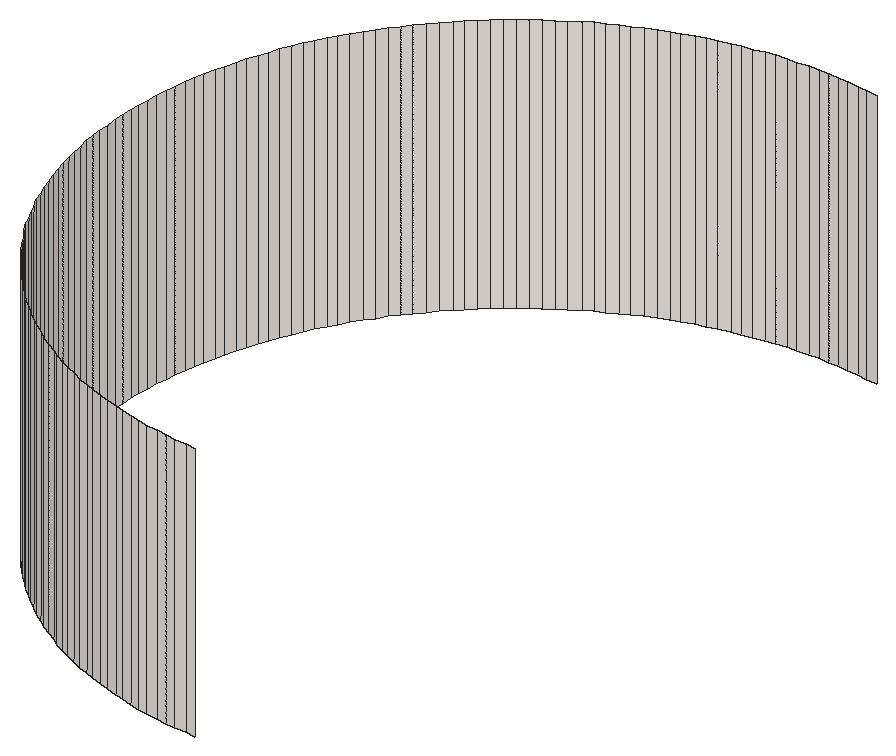
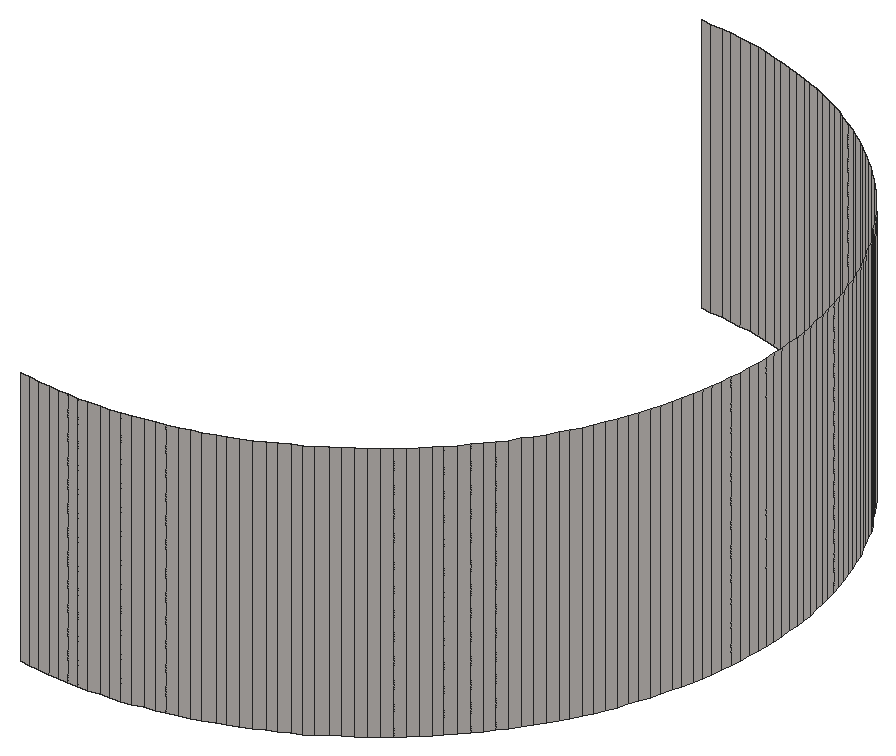
# SketchUp Ruby script. Lengths in inches.
U = 1.inch
M = Sketchup.active_model
def pt(a) = Geom::Point3d.new(a.map { |v| v * U })
def face(e, loops, mat)
  f = e.add_face(loops[0].map { |a| pt(a) })
  loops[1..].each { |l| e.add_face(l.map { |a| pt(a) }).erase! }
  f.material = f.back_material = mat if mat
  f
end
# faces: each face lists its corners as indices into pts; further lists are holes
def faces(e, pts, list, mat = nil) = list.each { |f| face(e, (f[0].is_a?(Array) ? f : [f]).map { |l| l.map { |i| pts[i] } }, mat) }
# xy, xz, yz: faces in a plane at the given z, y or x. An outline is a flat list of corners, or four numbers for a rectangle; further outlines are holes
def ring(l) = l.size == 4 ? [[l[0], l[1]], [l[2], l[1]], [l[2], l[3]], [l[0], l[3]]] : l.each_slice(2).to_a
def flat(e, list, mat, &to3) = list.each { |f| face(e, (f[0].is_a?(Array) ? f : [f]).map { |l| ring(l).map { |u, v| to3.(u, v) } }, mat) }
def xy(e, z, list, mat = nil) = flat(e, list, mat) { |x, y| [x, y, z] }
def xz(e, y, list, mat = nil) = flat(e, list, mat) { |x, z| [x, y, z] }
def yz(e, x, list, mat = nil) = flat(e, list, mat) { |y, z| [x, y, z] }
def lines(e, pts, list) = list.each { |a, b| e.add_line(pt(pts[a]), pt(pts[b])) }
# prism: a flat outline (further loops are holes) pulled along v
def prism(e, loops, v, mat = nil)
  f = face(e, loops, mat); d = Geom::Vector3d.new(v.map { |x| x * U })
  f.pushpull(f.normal.samedirection?(d) ? d.length : -d.length)
end
def box(e, o, s, mat = nil) = prism(e, [[o, [o[0] + s[0], o[1], o[2]], [o[0] + s[0], o[1] + s[1], o[2]], [o[0], o[1] + s[1], o[2]]]], [0, 0, s[2]], mat)
def at(x, y, z, deg = 0) = Geom::Transformation.translation(pt([x, y, z])) * Geom::Transformation.rotation(ORIGIN, Z_AXIS, deg.degrees)
def axes(o, x, y, z) = Geom::Transformation.new([*x, 0, *y, 0, *z, 0, *pt(o).to_a, 1])
def part(name) = M.definitions.add(name)
# library, detail: a bought-in or finely detailed component or shape, given as its bounding box
def library(name, o, s) = part(name).tap { |d| box(d.entities, o, s) }
def detail(e, o, s) = box(e.add_group.entities, o, s)
def put(e, d, t, mat = nil) = e.add_instance(d, t).tap { |i| i.material = mat if mat }
def group(e, t, mat = nil) = e.add_group.tap { |g| g.transformation = t; g.material = mat if mat }.entities
root = M.entities
M.materials.add("0001 AP 9436 AIR BREEZE").color = [243, 237, 232]
xz(root,40.51,[[23.75,106,23.83,108]],"0001 AP 9436 AIR BREEZE")
xz(root,46.49,[[23.7,106,23.78,108],[24.17,106,24.25,108]],"0001 AP 9436 AIR BREEZE")
xz(root,46.5,[[23.86,106,23.9375,108],[23.9375,106,24.02,108],[24.02,106,24.09,108]],"0001 AP 9436 AIR BREEZE")
yz(root,21,[[43.36,106,43.4375,108],[43.4375,106,43.52,108],[43.52,106,43.59,108]],"0001 AP 9436 AIR BREEZE")
yz(root,21.01,[[43.2,106,43.28,108],[43.67,106,43.75,108]],"0001 AP 9436 AIR BREEZE")
p = [[23.51,40.54,106],[23.4375,40.55,106],[23.4375,40.55,108],[23.51,40.54,108],[23.59,40.53,106],[23.59,40.53,108],
  [23.67,40.52,106],[23.67,40.52,108],[23.75,40.51,106],[23.75,40.51,108],[23.91,40.5,106],[23.83,40.51,106],
  [23.83,40.51,108],[23.91,40.5,108],[23.21,40.61,106],[23.13,40.63,106],[23.13,40.63,108],[23.21,40.61,108],
  [23.06,40.65,106],[23.06,40.65,108],[23.28,40.59,106],[23.28,40.59,108],[23.36,40.57,106],[23.36,40.57,108],
  [22.91,40.71,106],[22.84,40.73,106],[22.84,40.73,108],[22.91,40.71,108],[22.76,40.77,106],[22.76,40.77,108],
  [22.98,40.68,106],[22.98,40.68,108],[22.69,40.8,106],[22.625,40.83,106],[22.625,40.83,108],[22.69,40.8,108],
  [22.55,40.87,106],[22.55,40.87,108],[22.49,40.91,106],[22.42,40.95,106],[22.42,40.95,108],[22.49,40.91,108],
  [22.29,41.04,106],[22.22,41.08,106],[22.22,41.08,108],[22.29,41.04,108],[22.35,40.99,106],[22.35,40.99,108],
  [22.16,41.13,106],[22.1,41.18,106],[22.1,41.18,108],[22.16,41.13,108],[22.04,41.23,106],[22.04,41.23,108],
  [21.98,41.28,106],[21.98,41.28,108],[21.92,41.34,106],[21.92,41.34,108],[21.87,41.39,106],[21.87,41.39,108],
  [21.8125,41.45,106],[21.8125,41.45,108],[21.76,41.5,106],[21.76,41.5,108],[21.71,41.5625,106],[21.71,41.5625,108],
  [21.66,41.625,106],[21.61,41.6875,106],[21.61,41.6875,108],[21.66,41.625,108],[21.5625,41.75,106],[21.52,41.8125,106],
  [21.52,41.8125,108],[21.5625,41.75,108],[21.48,41.88,106],[21.48,41.88,108],[21.43,41.95,106],[21.43,41.95,108],
  [21.39,42.01,106],[21.39,42.01,108],[21.36,42.08,106],[21.36,42.08,108],[21.32,42.15,106],[21.32,42.15,108],
  [21.29,42.22,106],[21.29,42.22,108],[21.25,42.29,106],[21.25,42.29,108],[21.22,42.37,106],[21.22,42.37,108],
  [21.19,42.44,106],[21.19,42.44,108],[21.17,42.51,106],[21.17,42.51,108],[21.14,42.59,106],[21.14,42.59,108],
  [21.12,42.66,106],[21.12,42.66,108],[21.1,42.74,106],[21.1,42.74,108],[21.08,42.82,106],[21.08,42.82,108],
  [21.0625,42.89,106],[21.0625,42.89,108],[21.05,42.97,106],[21.05,42.97,108],[21.03,43.05,106],[21.03,43.05,108],
  [21.02,43.125,106],[21.02,43.125,108],[21.01,43.2,106],[21.01,43.2,108],[21.01,43.28,106],[21,43.36,106],
  [21,43.36,108],[21.01,43.28,108],[21,43.59,106],[21.01,43.67,106],[21.01,43.67,108],[21,43.59,108],
  [21.01,43.75,106],[21.02,43.83,106],[21.02,43.83,108],[21.01,43.75,108],[21.03,43.91,106],[21.03,43.91,108],
  [21.04,43.99,106],[21.04,43.99,108],[21.05,44.0625,106],[21.05,44.0625,108],[21.07,44.14,106],[21.07,44.14,108],
  [21.09,44.22,106],[21.09,44.22,108],[21.11,44.29,106],[21.11,44.29,108],[21.13,44.37,106],[21.13,44.37,108],
  [21.15,44.44,106],[21.15,44.44,108],[21.18,44.52,106],[21.18,44.52,108],[21.21,44.59,106],[21.21,44.59,108],
  [21.23,44.66,106],[21.23,44.66,108],[21.27,44.74,106],[21.27,44.74,108],[21.3,44.81,106],[21.3,44.81,108],
  [21.33,44.875,106],[21.33,44.875,108],[21.37,44.95,106],[21.37,44.95,108],[21.41,45.01,106],[21.41,45.01,108],
  [21.45,45.08,106],[21.45,45.08,108],[21.49,45.15,106],[21.49,45.15,108],[21.54,45.21,106],[21.54,45.21,108],
  [21.58,45.28,106],[21.58,45.28,108],[21.63,45.34,106],[21.63,45.34,108],[21.68,45.4,106],[21.68,45.4,108],
  [21.73,45.46,106],[21.73,45.46,108],[21.78,45.52,106],[21.78,45.52,108],[21.84,45.58,106],[21.84,45.58,108],
  [21.89,45.63,106],[21.89,45.63,108],[21.95,45.6875,106],[21.95,45.6875,108],[22,45.74,106],[22,45.74,108],
  [22.0625,45.79,106],[22.0625,45.79,108],[22.125,45.84,106],[22.125,45.84,108],[22.1875,45.89,106],[22.1875,45.89,108],
  [22.25,45.9375,106],[22.25,45.9375,108],[22.3125,45.98,106],[22.3125,45.98,108],[22.38,46.02,106],[22.38,46.02,108],
  [22.45,46.07,106],[22.45,46.07,108],[22.51,46.11,106],[22.51,46.11,108],[22.58,46.14,106],[22.58,46.14,108],
  [22.65,46.18,106],[22.65,46.18,108],[22.72,46.21,106],[22.72,46.21,108],[22.79,46.25,106],[22.79,46.25,108],
  [22.87,46.28,106],[22.87,46.28,108],[22.94,46.31,106],[22.94,46.31,108],[23.01,46.33,106],[23.01,46.33,108],
  [23.09,46.36,106],[23.09,46.36,108],[23.16,46.38,106],[23.16,46.38,108],[23.24,46.4,106],[23.24,46.4,108],
  [23.32,46.42,106],[23.32,46.42,108],[23.39,46.4375,106],[23.39,46.4375,108],[23.47,46.45,106],[23.47,46.45,108],
  [23.55,46.47,106],[23.55,46.47,108],[23.625,46.48,106],[23.625,46.48,108],[23.7,46.49,106],[23.7,46.49,108],
  [23.78,46.49,106],[23.86,46.5,106],[23.86,46.5,108],[23.78,46.49,108],[24.09,46.5,106],[24.17,46.49,106],
  [24.17,46.49,108],[24.09,46.5,108],[24.25,46.49,106],[24.33,46.48,106],[24.33,46.48,108],[24.25,46.49,108],
  [24.41,46.47,106],[24.41,46.47,108]]
faces(root,p,[[0,1,2,3],[4,0,3,5],[6,4,5,7],[8,6,7,9],[10,11,12,13],[14,15,16,17],[15,18,19,16],[20,14,17,21],
  [22,20,21,23],[1,22,23,2],[24,25,26,27],[25,28,29,26],[30,24,27,31],[18,30,31,19],[32,33,34,35],[33,36,37,34],
  [28,32,35,29],[38,39,40,41],[36,38,41,37],[42,43,44,45],[46,42,45,47],[39,46,47,40],[48,49,50,51],[43,48,51,44],
  [49,52,53,50],[52,54,55,53],[54,56,57,55],[56,58,59,57],[58,60,61,59],[60,62,63,61],[62,64,65,63],[66,67,68,69],
  [64,66,69,65],[70,71,72,73],[67,70,73,68],[71,74,75,72],[74,76,77,75],[76,78,79,77],[78,80,81,79],[80,82,83,81],
  [82,84,85,83],[84,86,87,85],[86,88,89,87],[88,90,91,89],[90,92,93,91],[92,94,95,93],[94,96,97,95],[96,98,99,97],
  [98,100,101,99],[100,102,103,101],[102,104,105,103],[104,106,107,105],[106,108,109,107],[108,110,111,109],[112,113,114,115],[116,117,118,119],
  [120,121,122,123],[121,124,125,122],[124,126,127,125],[126,128,129,127],[128,130,131,129],[130,132,133,131],[132,134,135,133],[134,136,137,135],
  [136,138,139,137],[138,140,141,139],[140,142,143,141],[142,144,145,143],[144,146,147,145],[146,148,149,147],[148,150,151,149],[150,152,153,151],
  [152,154,155,153],[154,156,157,155],[156,158,159,157],[158,160,161,159],[160,162,163,161],[162,164,165,163],[164,166,167,165],[166,168,169,167],
  [168,170,171,169],[170,172,173,171],[172,174,175,173],[174,176,177,175],[176,178,179,177],[178,180,181,179],[180,182,183,181],[182,184,185,183],
  [184,186,187,185],[186,188,189,187],[188,190,191,189],[190,192,193,191],[192,194,195,193],[194,196,197,195],[196,198,199,197],[198,200,201,199],
  [200,202,203,201],[202,204,205,203],[204,206,207,205],[206,208,209,207],[208,210,211,209],[210,212,213,211],[212,214,215,213],[214,216,217,215],
  [216,218,219,217],[218,220,221,219],[220,222,223,221],[222,224,225,223],[224,226,227,225],[228,229,230,231],[232,233,234,235],[236,237,238,239],
  [237,240,241,238]],"0001 AP 9436 AIR BREEZE")
